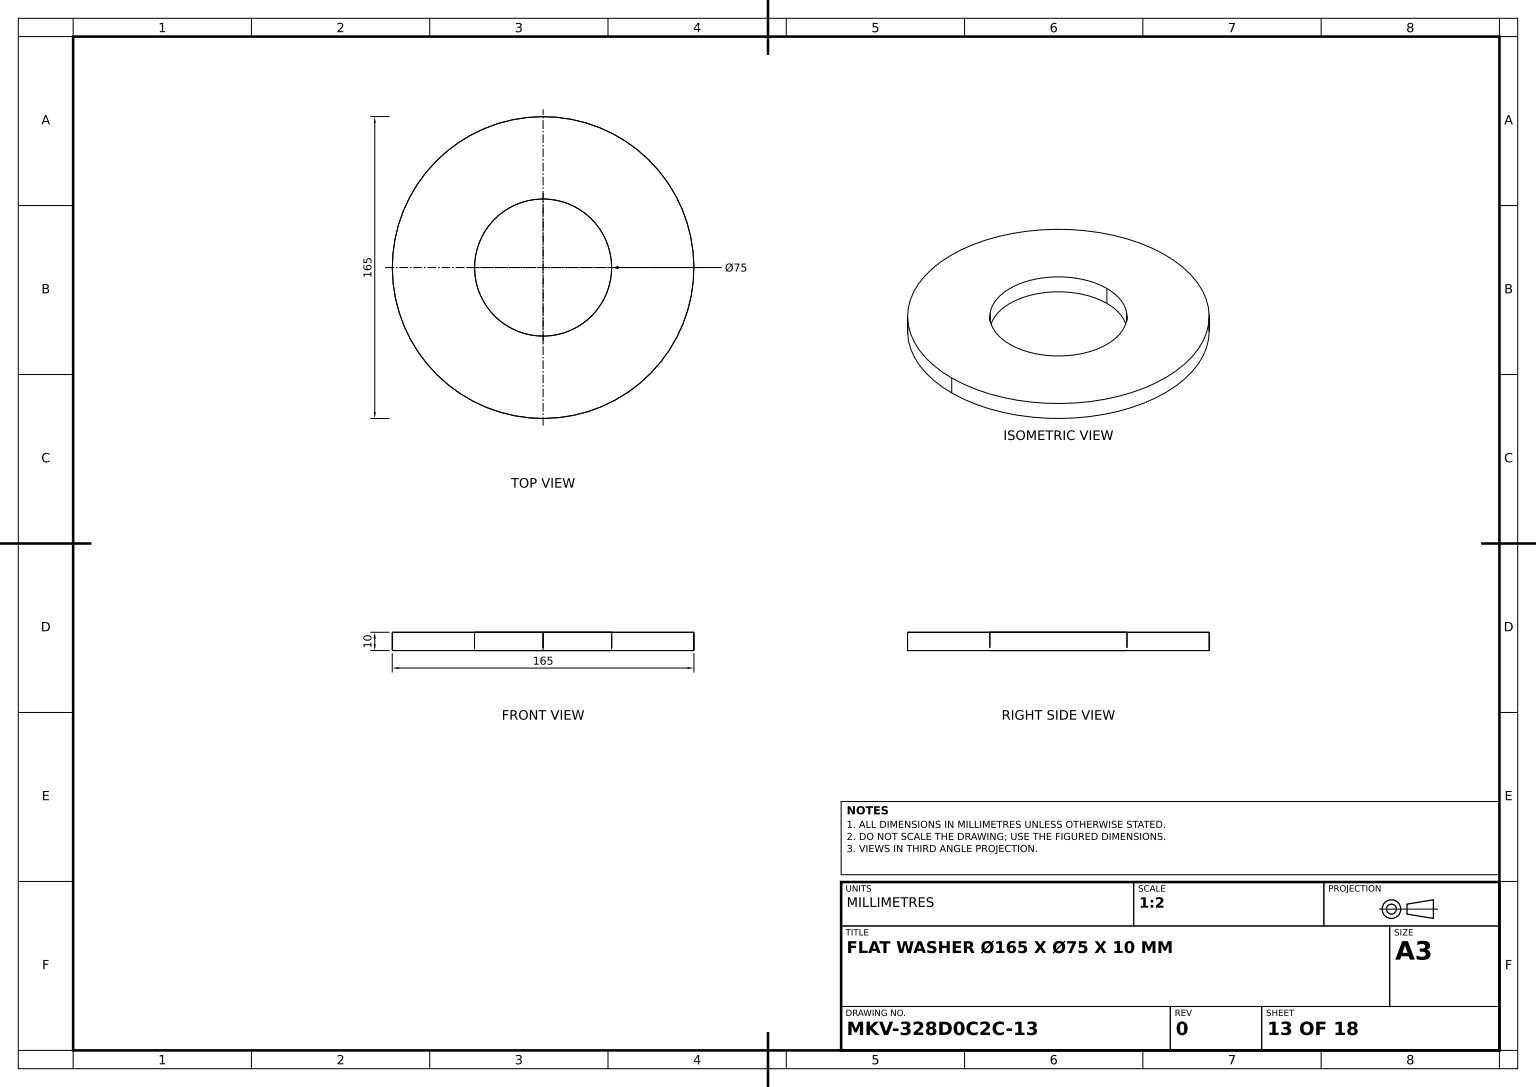
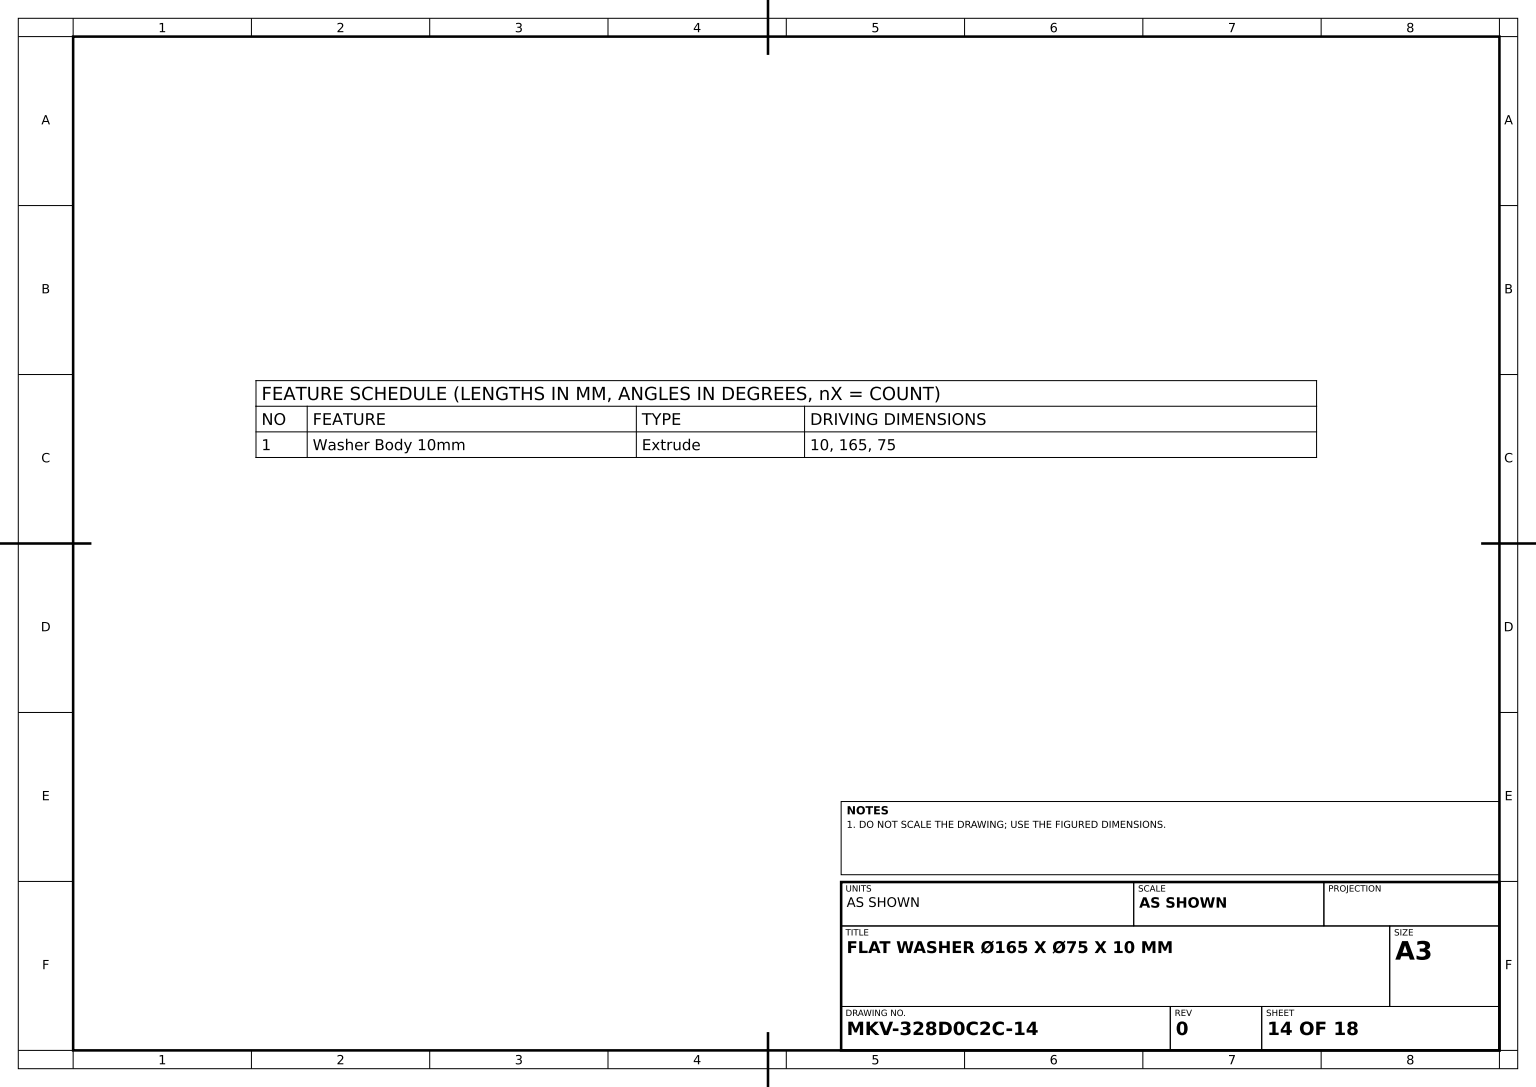
ISO-10303-21;
HEADER;
FILE_DESCRIPTION((''),'2;1');
FILE_NAME('','',(''),(''),'','','');
FILE_SCHEMA(('AUTOMOTIVE_DESIGN'));
ENDSEC;
DATA;
#1=APPLICATION_CONTEXT('');
#2=PRODUCT_CONTEXT('',#1,'mechanical');
#3=PRODUCT('','','',(#2));
#4=PRODUCT_DEFINITION_FORMATION('','',#3);
#5=PRODUCT_DEFINITION_CONTEXT('',#1,'design');
#6=PRODUCT_DEFINITION('','',#4,#5);
#7=PRODUCT_DEFINITION_SHAPE('','',#6);
#8=(LENGTH_UNIT()NAMED_UNIT(*)SI_UNIT(.MILLI.,.METRE.));
#9=(NAMED_UNIT(*)PLANE_ANGLE_UNIT()SI_UNIT($,.RADIAN.));
#10=(NAMED_UNIT(*)SI_UNIT($,.STERADIAN.)SOLID_ANGLE_UNIT());
#11=UNCERTAINTY_MEASURE_WITH_UNIT(LENGTH_MEASURE(1.E-05),#8,'distance_accuracy_value','');
#12=(GEOMETRIC_REPRESENTATION_CONTEXT(3)GLOBAL_UNCERTAINTY_ASSIGNED_CONTEXT((#11))GLOBAL_UNIT_ASSIGNED_CONTEXT((#8,#9,#10))REPRESENTATION_CONTEXT('',''));
#13=CARTESIAN_POINT('',(0.,10.,37.5));
#14=VERTEX_POINT('',#13);
#15=CARTESIAN_POINT('',(0.,10.,-37.5));
#16=VERTEX_POINT('',#15);
#17=CARTESIAN_POINT('',(0.,10.,0.));
#18=DIRECTION('',(0.,1.,0.));
#19=DIRECTION('',(0.,0.,1.));
#20=AXIS2_PLACEMENT_3D('',#17,#18,#19);
#21=CIRCLE('',#20,37.5);
#22=EDGE_CURVE('',#14,#16,#21,.T.);
#23=ORIENTED_EDGE('',*,*,#22,.T.);
#24=CARTESIAN_POINT('',(0.,0.,-37.5));
#25=VERTEX_POINT('',#24);
#26=DIRECTION('',(0.,-1.,0.));
#27=VECTOR('',#26,1000.);
#28=LINE('',#15,#27);
#29=EDGE_CURVE('',#16,#25,#28,.T.);
#30=ORIENTED_EDGE('',*,*,#29,.T.);
#31=CARTESIAN_POINT('',(0.,0.,37.5));
#32=VERTEX_POINT('',#31);
#33=CARTESIAN_POINT('',(0.,0.,0.));
#34=AXIS2_PLACEMENT_3D('',#33,#18,#19);
#35=CIRCLE('',#34,37.5);
#36=EDGE_CURVE('',#32,#25,#35,.T.);
#37=ORIENTED_EDGE('',*,*,#36,.F.);
#38=LINE('',#13,#27);
#39=EDGE_CURVE('',#14,#32,#38,.T.);
#40=ORIENTED_EDGE('',*,*,#39,.F.);
#41=EDGE_LOOP('',(#23,#30,#37,#40));
#42=FACE_OUTER_BOUND('',#41,.T.);
#43=DIRECTION('',(0.,0.,-1.));
#44=AXIS2_PLACEMENT_3D('',#17,#26,#43);
#45=CYLINDRICAL_SURFACE('',#44,37.5);
#46=ADVANCED_FACE('',(#42),#45,.F.);
#47=CARTESIAN_POINT('',(0.,0.,-82.5));
#48=VERTEX_POINT('',#47);
#49=CARTESIAN_POINT('',(0.,0.,82.5));
#50=VERTEX_POINT('',#49);
#51=CIRCLE('',#34,82.5);
#52=EDGE_CURVE('',#48,#50,#51,.T.);
#53=ORIENTED_EDGE('',*,*,#52,.T.);
#54=CARTESIAN_POINT('',(0.,10.,82.5));
#55=VERTEX_POINT('',#54);
#56=LINE('',#54,#27);
#57=EDGE_CURVE('',#55,#50,#56,.T.);
#58=ORIENTED_EDGE('',*,*,#57,.F.);
#59=CARTESIAN_POINT('',(0.,10.,-82.5));
#60=VERTEX_POINT('',#59);
#61=CIRCLE('',#20,82.5);
#62=EDGE_CURVE('',#60,#55,#61,.T.);
#63=ORIENTED_EDGE('',*,*,#62,.F.);
#64=LINE('',#59,#27);
#65=EDGE_CURVE('',#60,#48,#64,.T.);
#66=ORIENTED_EDGE('',*,*,#65,.T.);
#67=EDGE_LOOP('',(#53,#58,#63,#66));
#68=FACE_OUTER_BOUND('',#67,.T.);
#69=CYLINDRICAL_SURFACE('',#44,82.5);
#70=ADVANCED_FACE('',(#68),#69,.T.);
#71=EDGE_CURVE('',#16,#14,#21,.T.);
#72=ORIENTED_EDGE('',*,*,#71,.T.);
#73=ORIENTED_EDGE('',*,*,#39,.T.);
#74=EDGE_CURVE('',#25,#32,#35,.T.);
#75=ORIENTED_EDGE('',*,*,#74,.F.);
#76=ORIENTED_EDGE('',*,*,#29,.F.);
#77=EDGE_LOOP('',(#72,#73,#75,#76));
#78=FACE_OUTER_BOUND('',#77,.T.);
#79=ADVANCED_FACE('',(#78),#45,.F.);
#80=EDGE_CURVE('',#55,#60,#61,.T.);
#81=ORIENTED_EDGE('',*,*,#80,.T.);
#82=ORIENTED_EDGE('',*,*,#62,.T.);
#83=EDGE_LOOP('',(#81,#82));
#84=FACE_OUTER_BOUND('',#83,.T.);
#85=ORIENTED_EDGE('',*,*,#22,.F.);
#86=ORIENTED_EDGE('',*,*,#71,.F.);
#87=EDGE_LOOP('',(#85,#86));
#88=FACE_BOUND('',#87,.T.);
#89=PLANE('',#20);
#90=ADVANCED_FACE('',(#84,#88),#89,.T.);
#91=ORIENTED_EDGE('',*,*,#52,.F.);
#92=EDGE_CURVE('',#50,#48,#51,.T.);
#93=ORIENTED_EDGE('',*,*,#92,.F.);
#94=EDGE_LOOP('',(#91,#93));
#95=FACE_OUTER_BOUND('',#94,.T.);
#96=ORIENTED_EDGE('',*,*,#74,.T.);
#97=ORIENTED_EDGE('',*,*,#36,.T.);
#98=EDGE_LOOP('',(#96,#97));
#99=FACE_BOUND('',#98,.T.);
#100=PLANE('',#34);
#101=ADVANCED_FACE('',(#95,#99),#100,.F.);
#102=ORIENTED_EDGE('',*,*,#57,.T.);
#103=ORIENTED_EDGE('',*,*,#92,.T.);
#104=ORIENTED_EDGE('',*,*,#65,.F.);
#105=ORIENTED_EDGE('',*,*,#80,.F.);
#106=EDGE_LOOP('',(#102,#103,#104,#105));
#107=FACE_OUTER_BOUND('',#106,.T.);
#108=ADVANCED_FACE('',(#107),#69,.T.);
#109=CLOSED_SHELL('',(#46,#70,#79,#90,#101,#108));
#110=MANIFOLD_SOLID_BREP('',#109);
#111=ADVANCED_BREP_SHAPE_REPRESENTATION('',(#110),#12);
#112=SHAPE_DEFINITION_REPRESENTATION(#7,#111);
ENDSEC;
END-ISO-10303-21;
